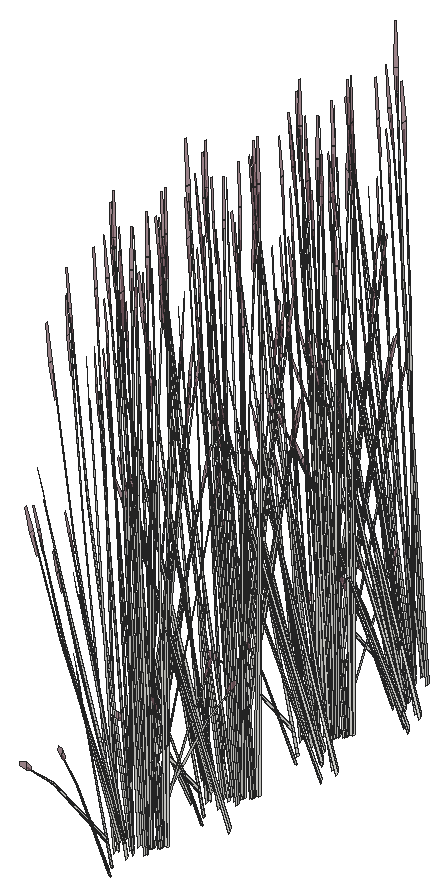
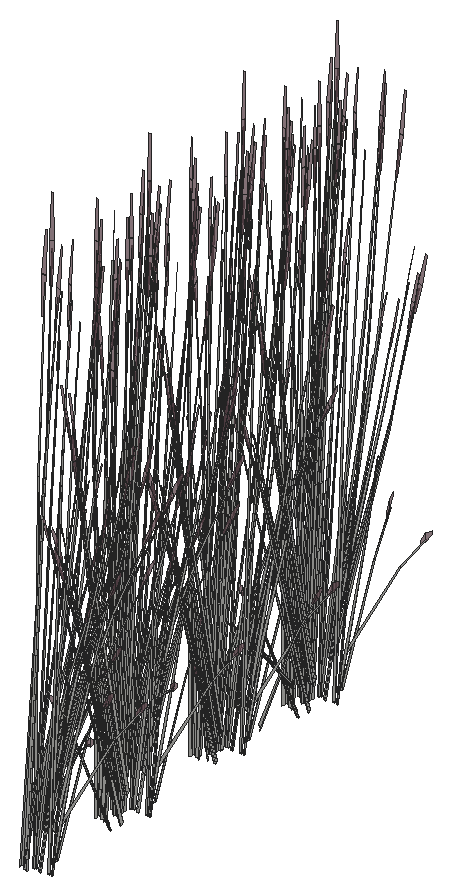
# SketchUp Ruby script. Lengths in inches.
U = 1.inch
M = Sketchup.active_model
def pt(a) = Geom::Point3d.new(a.map { |v| v * U })
def face(e, loops, mat)
  f = e.add_face(loops[0].map { |a| pt(a) })
  loops[1..].each { |l| e.add_face(l.map { |a| pt(a) }).erase! }
  f.material = f.back_material = mat if mat
  f
end
# faces: each face lists its corners as indices into pts; further lists are holes
def faces(e, pts, list, mat = nil) = list.each { |f| face(e, (f[0].is_a?(Array) ? f : [f]).map { |l| l.map { |i| pts[i] } }, mat) }
# xy, xz, yz: faces in a plane at the given z, y or x. An outline is a flat list of corners, or four numbers for a rectangle; further outlines are holes
def ring(l) = l.size == 4 ? [[l[0], l[1]], [l[2], l[1]], [l[2], l[3]], [l[0], l[3]]] : l.each_slice(2).to_a
def flat(e, list, mat, &to3) = list.each { |f| face(e, (f[0].is_a?(Array) ? f : [f]).map { |l| ring(l).map { |u, v| to3.(u, v) } }, mat) }
def xy(e, z, list, mat = nil) = flat(e, list, mat) { |x, y| [x, y, z] }
def xz(e, y, list, mat = nil) = flat(e, list, mat) { |x, z| [x, y, z] }
def yz(e, x, list, mat = nil) = flat(e, list, mat) { |y, z| [x, y, z] }
def lines(e, pts, list) = list.each { |a, b| e.add_line(pt(pts[a]), pt(pts[b])) }
# prism: a flat outline (further loops are holes) pulled along v
def prism(e, loops, v, mat = nil)
  f = face(e, loops, mat); d = Geom::Vector3d.new(v.map { |x| x * U })
  f.pushpull(f.normal.samedirection?(d) ? d.length : -d.length)
end
def box(e, o, s, mat = nil) = prism(e, [[o, [o[0] + s[0], o[1], o[2]], [o[0] + s[0], o[1] + s[1], o[2]], [o[0], o[1] + s[1], o[2]]]], [0, 0, s[2]], mat)
def at(x, y, z, deg = 0) = Geom::Transformation.translation(pt([x, y, z])) * Geom::Transformation.rotation(ORIGIN, Z_AXIS, deg.degrees)
def axes(o, x, y, z) = Geom::Transformation.new([*x, 0, *y, 0, *z, 0, *pt(o).to_a, 1])
def part(name) = M.definitions.add(name)
# library, detail: a bought-in or finely detailed component or shape, given as its bounding box
def library(name, o, s) = part(name).tap { |d| box(d.entities, o, s) }
def detail(e, o, s) = box(e.add_group.entities, o, s)
def put(e, d, t, mat = nil) = e.add_instance(d, t).tap { |i| i.material = mat if mat }
def group(e, t, mat = nil) = e.add_group.tap { |g| g.transformation = t; g.material = mat if mat }.entities
root = M.entities
M.materials.add("LightPink_Translucent").color = [144, 107, 117]
M.materials["LightPink_Translucent"].alpha = 0.75
c1 = part("blade")
p = [[2.15,0.21,22],[0,0.17,0],[0.09,0.45,0],[2.18,0.31,22],[2.29,0.31,22],[0.38,0.45,0],
  [2.48,0.24,33],[2.49,0.24,33],[2.48,0.22,33]]
faces(c1.entities,p,[[0,1,2,3],[4,5,2,3],[6,3,4,7],[8,0,3,6]])
c2 = part("seeds")
p = [[0.3,-0.1,1.38],[-0.01,-0.03,1.59],[-0.01,-0.03,0.03],[0.14,-0.07,-0.07],[0.29,-0.03,3],[0.15,0.01,3.11]]
faces(c2.entities,p,[[0,1,2,3],[1,0,4,5]],"LightPink_Translucent")
c3 = part("blade with seeds")
put(c3.entities,c1,at(0,0,0))
put(c3.entities,c2,axes([2.4,0.25,30.99],[1.5799,-0.05474,1.17369],[-0.12525,1.92788,0.29478],[-0.07173,-0.02425,1.56792]))
put(root,c3,axes([403.09,8.77,-7.61],[-0.07822,-0.07621,1.62908],[-0.52201,0.04832,-0.25764],[-0.08331,-0.18228,0.13065]))
put(root,c3,axes([403.63,10.06,-7.36],[-0.24409,-0.44196,-0.66157],[0.50245,-0.2463,0.07984],[-0.05708,-0.21354,0.93586]))
put(root,c3,axes([403.21,9.08,-10.61],[-0.08578,0.01958,1.6421],[-0.47437,-0.22044,-0.25086],[0.00796,-0.18387,0.2797]))
put(root,c3,axes([403.68,9.68,-7.78],[0.15418,-0.41799,-0.32977],[0.44981,0.12192,0.42575],[-0.04124,-0.16829,0.81462]))
put(root,c3,axes([403.45,9.97,-7.64],[-0.50273,-0.13626,-0.47583],[0.17232,-0.46717,-0.36857],[-0.0461,-0.18809,0.91046]))
put(root,c3,axes([403.88,9.95,-7.3125],[-0.50045,0.25306,-0.11324],[-0.24593,-0.44915,-0.62851],[-0.06603,-0.18927,0.95501]))
put(root,c3,axes([403.87,9.74,-7.6],[0.37684,-0.18473,0.05988],[0.18445,0.33686,0.47138],[-0.03639,-0.14849,0.71878]))
put(root,c3,axes([402.51,11.72,-10.05],[-0.21003,-0.55738,-0.65031],[0.60499,-0.20074,-0.17068],[-0.02321,-0.18874,1.43544]))
put(root,c3,axes([403.73,10.12,-7.3],[-0.15418,0.41799,0.32977],[-0.44981,-0.12192,-0.42575],[-0.04124,-0.16829,0.81462]))
put(root,c3,axes([403.125,9.46,-10.02],[-0.35341,0.31182,-0.03625],[-0.32382,-0.34152,-0.16435],[-0.0228,-0.09677,0.54209]))
put(root,c3,axes([401.27,11.64,-10.12],[0,-0.54355,-0.46235],[0.57217,0,0],[0,-0.1238,1.46668]))
put(root,c3,axes([402.82,11.86,-9.94],[0.24813,-0.48978,-0.41661],[0.51557,0.23571,0.2005],[0,-0.1129,1.33761]))
put(root,c3,axes([401.51,11.65,-10.11],[0.35699,-0.33913,-0.28847],[0.35699,0.33913,0.28847],[0,-0.10923,1.29413]))
put(root,c3,axes([402.76,12.27,-9.52],[-0.57594,-0.25935,-0.27094],[0.27732,-0.5474,-0.46562],[-0.0181,-0.1344,1.4872]))
put(root,c3,axes([401.51,12.14,-9.69],[0,0.54355,0.46235],[-0.57217,0,0],[0,-0.1238,1.46668]))
put(root,c3,axes([402.93,11.9375,-9.8],[0.22235,0.6078,0.42607],[-0.63531,0.21135,0.16719],[0.00776,-0.11168,1.47927]))
put(root,c3,axes([402.82,12.42,-9.47],[-0.24813,0.48978,0.41661],[-0.51557,-0.23571,-0.2005],[0,-0.1129,1.33761]))
put(root,c3,axes([403.89,12.48,-9.86],[-0.47569,-0.46784,-0.05709],[0.47598,-0.46812,0],[-0.01661,-0.01634,1.63492]))
put(root,c3,axes([402.98,12.53,-9.8],[0.64638,0.11452,0.42607],[-0.13155,0.64678,0.16719],[-0.09446,-0.06245,1.47927]))
put(root,c3,axes([402.64,13.57,-9.7],[0.54955,-0.14427,0.16428],[0.1357,0.53689,0.32672],[-0.04901,-0.07823,1.49371]))
put(root,c3,axes([403.46,13.44,-9.95],[-0.16686,-0.46861,0],[0.47648,-0.16411,0],[0,0,1.4375]))
put(root,c3,axes([403.14,13,-9.5625],[-0.09866,0.48509,0.13483],[-0.48202,-0.0842,-0.38503],[-0.08772,-0.04981,1.18024]))
put(root,c3,axes([404.27,13.6,-9.7],[0.14774,-0.54019,0.16428],[0.54062,0.15287,0.32672],[-0.09339,0.00263,1.49371]))
put(root,c3,axes([403.34,13.65,-9.95],[-0.51557,-0.24403,0],[0.24813,-0.50705,0],[0,0,1.51513]))
put(root,c3,axes([404.01,12.64,-9.47],[0.55535,-0.03355,0.41661],[0.05022,0.55698,-0.2005],[-0.09942,0.05645,1.33761]))
put(root,c3,axes([404.13,14.2,-9.96],[-0.31576,-0.54657,-0.04789],[0.53494,-0.30375,0.48057],[-0.13182,0.05204,1.52373]))
put(root,c3,axes([404.02,12.88,-9.5625],[0.37783,0.32657,0.13483],[-0.31516,0.36844,-0.38503],[-0.08772,0.04981,1.18024]))
put(root,c3,axes([404.42,13.89,-9.69],[0.47863,-0.27177,0.46235],[0.28609,0.48733,0],[-0.10901,0.0619,1.46668]))
put(root,c3,axes([403.99,14.13,-10.11],[-0.47712,-0.13449,-0.28847],[0.12013,-0.47362,0.28847],[-0.09619,0.05462,1.29413]))
put(root,c3,axes([403.91,12.76,-9.52],[0.05959,0.62022,-0.27094],[-0.62068,0.0375,-0.46562],[-0.1093,0.08261,1.4872]))
put(root,c3,axes([404.13,12.52,-9.94],[-0.24813,0.48978,-0.41661],[-0.51557,-0.23571,0.2005],[0,0.1129,1.33761]))
put(root,c3,axes([404.15,13.92,-9.83],[0.64025,0.17667,0.2864],[-0.16018,0.63149,-0.33981],[-0.10597,0.07904,1.53541]))
put(root,c3,axes([404.1,14.35,-10.12],[-0.47863,0.27177,-0.46235],[-0.28609,-0.48733,0],[-0.10901,0.0619,1.46668]))
put(root,c3,axes([403.7,19.37,-7.61],[-0.07822,-0.07621,1.62908],[-0.52201,0.04832,-0.25764],[-0.08331,-0.18228,0.13065]))
put(root,c3,axes([404.25,20.66,-7.36],[-0.24409,-0.44196,-0.66157],[0.50245,-0.2463,0.07984],[-0.05708,-0.21354,0.93586]))
put(root,c3,axes([408.66,16.62,-8.39],[0.21212,-0.01231,1.59586],[-0.14072,0.53355,0.12904],[-0.3023,-0.033,0.68222]))
put(root,c3,axes([403.83,19.68,-10.61],[-0.08578,0.01958,1.6421],[-0.47437,-0.22044,-0.25086],[0.00796,-0.18387,0.2797]))
put(root,c3,axes([401.94,13.68,-7.3],[0.34603,-0.28618,0.32977],[0.32756,0.32677,-0.42575],[-0.04984,0.16603,0.81462]))
put(root,c3,axes([404.54,14.26,-9.79],[0.31974,0.54466,0],[-0.53494,0.30375,-0.48057],[-0.12184,0.06918,1.52448]))
put(root,c3,axes([404.26,12.11,-9.35],[-0.01397,-0.51177,1.31553],[0.63227,0.13266,0.557],[-0.14954,0.28003,1.24175]))
put(root,c3,axes([404.07,20.57,-7.64],[-0.50273,-0.13626,-0.47583],[0.17232,-0.46717,-0.36857],[-0.0461,-0.18809,0.91046]))
put(root,c3,axes([403.07,20.27,-7.26],[0.56969,-0.13971,0.50064],[0.09887,0.54803,0.4128],[-0.13398,-0.16152,1.03595]))
put(root,c3,axes([404.5,20.54,-7.3125],[-0.50045,0.25306,-0.11324],[-0.24593,-0.44915,-0.62851],[-0.06603,-0.18927,0.95501]))
put(root,c3,axes([402.77,14.53,-7.6],[-0.37684,0.18473,0.05988],[-0.18445,-0.33686,0.47138],[0.03639,0.14849,0.71878]))
put(root,c3,axes([402.51,19.78,-9.42],[0.26677,0.18918,1.06958],[-0.38851,0.11372,0.78586],[-0.08313,-0.14539,0.23558]))
put(root,c3,axes([401.72,13.76,-6.97],[0.56206,0.02693,-0.12569],[-0.01536,0.50991,-0.69765],[-0.03904,0.19638,1.06006]))
put(root,c3,axes([402.91,14.5,-7.28],[-0.50393,-0.1421,0.49617],[0.17232,-0.46717,0.40911],[0.03028,0.18372,1.0267]))
put(root,c3,axes([402.85,14.43,-10.61],[0.08277,-0.02958,1.6421],[0.49786,0.16279,-0.25086],[0.01456,0.18348,0.2797]))
put(root,c3,axes([402.11,13.95,-7.34],[0.3661,0.36521,-0.52818],[-0.38674,0.31985,-0.40911],[-0.0557,0.18556,1.01061]))
put(root,c3,axes([403.2,20.39,-7.6],[0.23243,-0.34529,0.05988],[0.331,0.20103,0.47138],[-0.10701,-0.1107,0.71878]))
put(root,c3,axes([401.71,14.5,-9.37],[0.46459,-0.09625,0.0606],[0.10681,0.38778,-0.80367],[-0.02945,0.1963,0.72038]))
put(root,c3,axes([403.125,22.32,-10.05],[-0.21003,-0.55738,-0.65031],[0.60499,-0.20074,-0.17068],[-0.02321,-0.18874,1.43544]))
put(root,c3,axes([402.96,14.6,-7.78],[-0.15418,0.41799,-0.32977],[-0.44981,-0.12192,0.42575],[0.04124,0.16829,0.81462]))
put(root,c3,axes([404.35,20.72,-7.3],[-0.15418,0.41799,0.32977],[-0.44981,-0.12192,-0.42575],[-0.04124,-0.16829,0.81462]))
put(root,c3,axes([402.52,13.43,-8.39],[-0.01252,-0.20862,1.59586],[0.54251,0.1384,0.12904],[-0.03356,0.2973,0.68222]))
put(root,c3,axes([403.74,20.06,-10.02],[-0.35341,0.31182,-0.03625],[-0.32382,-0.34152,-0.16435],[-0.0228,-0.09677,0.54209]))
put(root,c3,axes([402.65,15.34,-7.61],[0.06483,0.08753,1.62908],[0.52315,0.03439,-0.25764],[0.05261,0.19303,0.13065]))
put(root,c3,axes([401.89,22.24,-10.12],[0,-0.54355,-0.46235],[0.57217,0,0],[0,-0.1238,1.46668]))
put(root,c3,axes([402.13,22.25,-10.11],[0.35699,-0.33913,-0.28847],[0.35699,0.33913,0.28847],[0,-0.10923,1.29413]))
put(root,c3,axes([403.38,22.87,-9.52],[-0.57594,-0.25935,-0.27094],[0.27732,-0.5474,-0.46562],[-0.0181,-0.1344,1.4872]))
put(root,c3,axes([403.53,23.44,-9.73],[0.13555,-0.64407,-0.21817],[0.64269,0.11227,0.47743],[-0.1123,-0.08895,1.45677]))
put(root,c3,axes([402.13,22.74,-9.69],[0,0.54355,0.46235],[-0.57217,0,0],[0,-0.1238,1.46668]))
put(root,c3,axes([403.48,23.18,-9.94],[-0.30722,-0.45622,-0.41661],[0.46535,-0.32126,0.2005],[-0.09942,-0.05645,1.33761]))
put(root,c3,axes([403.43,23.02,-9.47],[-0.24813,0.48978,0.41661],[-0.51557,-0.23571,-0.2005],[0,-0.1129,1.33761]))
put(root,c3,axes([404.51,23.08,-9.86],[-0.47569,-0.46784,-0.05709],[0.47598,-0.46812,0],[-0.01661,-0.01634,1.63492]))
put(root,c3,axes([403.6,23.13,-9.8],[0.64638,0.11452,0.42607],[-0.13155,0.64678,0.16719],[-0.09446,-0.06245,1.47927]))
put(root,c3,axes([403.25,24.17,-9.7],[0.54955,-0.14427,0.16428],[0.1357,0.53689,0.32672],[-0.04901,-0.07823,1.49371]))
put(root,c3,axes([403.76,23.59,-9.5625],[-0.09866,0.48509,0.13483],[-0.48202,-0.0842,-0.38503],[-0.08772,-0.04981,1.18024]))
put(root,c3,axes([404.89,24.2,-9.7],[0.14774,-0.54019,0.16428],[0.54062,0.15287,0.32672],[-0.09339,0.00263,1.49371]))
put(root,c3,axes([403.96,24.25,-9.95],[-0.51557,-0.24403,0],[0.24813,-0.50705,0],[0,0,1.51513]))
put(root,c3,axes([404.39,23.6,-9.7],[-0.49938,-0.43748,-0.23459],[0.42021,-0.49126,0.51337],[-0.13447,0.05118,1.56642]))
put(root,c3,axes([403.07,24.44,-9.69],[0.47863,0.27177,0.46235],[-0.28609,0.48733,0],[-0.10901,-0.0619,1.46668]))
put(root,c3,axes([404.63,23.24,-9.47],[0.55535,-0.03355,0.41661],[0.05022,0.55698,-0.2005],[-0.09942,0.05645,1.33761]))
put(root,c3,axes([404.14,23.51,-9.94],[-0.55535,0.03355,-0.41661],[-0.05022,-0.55698,0.2005],[-0.09942,0.05645,1.33761]))
put(root,c3,axes([404.75,24.8,-9.96],[-0.31576,-0.54657,-0.04789],[0.53494,-0.30375,0.48057],[-0.13182,0.05204,1.52373]))
put(root,c3,axes([404.64,23.48,-9.5625],[0.37783,0.32657,0.13483],[-0.31516,0.36844,-0.38503],[-0.08772,0.04981,1.18024]))
put(root,c3,axes([404.61,24.73,-10.11],[-0.47712,-0.13449,-0.28847],[0.12013,-0.47362,0.28847],[-0.09619,0.05462,1.29413]))
put(root,c3,axes([404.53,23.36,-9.52],[0.05959,0.62022,-0.27094],[-0.62068,0.0375,-0.46562],[-0.1093,0.08261,1.4872]))
put(root,c3,axes([404.77,24.52,-9.83],[0.64025,0.17667,0.2864],[-0.16018,0.63149,-0.33981],[-0.10597,0.07904,1.53541]))
put(root,c3,axes([404.72,24.95,-10.12],[-0.47863,0.27177,-0.46235],[-0.28609,-0.48733,0],[-0.10901,0.0619,1.46668]))
put(root,c3,axes([402.5625,24.28,-7.3],[0.34603,-0.28618,0.32977],[0.32756,0.32677,-0.42575],[-0.04984,0.16603,0.81462]))
put(root,c3,axes([405.15,24.86,-9.79],[0.31974,0.54466,0],[-0.53494,0.30375,-0.48057],[-0.12184,0.06918,1.52448]))
put(root,c3,axes([404.88,22.71,-9.35],[-0.01397,-0.51177,1.31553],[0.63227,0.13266,0.557],[-0.14954,0.28003,1.24175]))
put(root,c3,axes([407.875,28.96,-9.59],[0.09985,0.15133,1.33163],[-0.23008,0.41134,-0.28638],[-0.23625,-0.09832,0.56934]))
put(root,c3,axes([408.29,28.82,-7.36],[-0.51122,-0.01309,-0.66157],[0.03434,-0.5511,0.07984],[-0.21658,-0.05816,0.93586]))
put(root,c3,axes([403.33,31.36,-7.61],[-0.07822,-0.07621,1.62908],[-0.52201,0.04832,-0.25764],[-0.08331,-0.18228,0.13065]))
put(root,c3,axes([403.39,25.13,-7.6],[-0.37684,0.18473,0.05988],[-0.18445,-0.33686,0.47138],[0.03639,0.14849,0.71878]))
put(root,c3,axes([402.34,24.36,-6.97],[0.56206,0.02693,-0.12569],[-0.01536,0.50991,-0.69765],[-0.03904,0.19638,1.06006]))
put(root,c3,axes([403.88,32.64,-7.36],[-0.24409,-0.44196,-0.66157],[0.50245,-0.2463,0.07984],[-0.05708,-0.21354,0.93586]))
put(root,c3,axes([403.53,25.1,-7.28],[-0.50393,-0.1421,0.49617],[0.17232,-0.46717,0.40911],[0.03028,0.18372,1.0267]))
put(root,c3,axes([402.6,25.8,-9.42],[-0.01324,-0.32319,1.06958],[0.33072,0.23052,0.78586],[-0.06504,0.15405,0.23558]))
put(root,c3,axes([403.46,31.66,-10.61],[-0.08578,0.01958,1.6421],[-0.47437,-0.22044,-0.25086],[0.00796,-0.18387,0.2797]))
put(root,c3,axes([402.73,24.55,-7.34],[0.3661,0.36521,-0.52818],[-0.38674,0.31985,-0.40911],[-0.0557,0.18556,1.01061]))
put(root,c3,axes([402.33,25.1,-9.37],[0.46459,-0.09625,0.0606],[0.10681,0.38778,-0.80367],[-0.02945,0.1963,0.72038]))
put(root,c3,axes([403.92,32.27,-7.78],[0.15418,-0.41799,-0.32977],[0.44981,0.12192,0.42575],[-0.04124,-0.16829,0.81462]))
put(root,c3,axes([407.65,29.32,-8.39],[0.21212,-0.01231,1.59586],[-0.14072,0.53355,0.12904],[-0.3023,-0.033,0.68222]))
put(root,c3,axes([403.69,32.55,-7.64],[-0.50273,-0.13626,-0.47583],[0.17232,-0.46717,-0.36857],[-0.0461,-0.18809,0.91046]))
put(root,c3,axes([402.61,24.39,-7.03],[-0.01331,0.50278,-0.73435],[-0.56035,-0.03377,0.08862],[-0.05914,0.213,1.03881]))
put(root,c3,axes([403.14,24.03,-8.39],[-0.01252,-0.20862,1.59586],[0.54251,0.1384,0.12904],[-0.03356,0.2973,0.68222]))
put(root,c3,axes([404.125,32.53,-7.3125],[-0.50045,0.25306,-0.11324],[-0.24593,-0.44915,-0.62851],[-0.06603,-0.18927,0.95501]))
put(root,c3,axes([402.75,34.3,-10.05],[-0.21003,-0.55738,-0.65031],[0.60499,-0.20074,-0.17068],[-0.02321,-0.18874,1.43544]))
put(root,c3,axes([402.42,25.09,-8.87],[0.01124,-0.2806,1.43727],[0.50537,0.14821,0.19862],[-0.04379,0.29905,0.67868]))
put(root,c3,axes([407.47,29.78,-7.78],[-0.42502,-0.15163,-0.32977],[0.12396,-0.44238,0.42575],[-0.17112,0.04056,0.81462]))
put(root,c3,axes([403.97,32.71,-7.3],[-0.15418,0.41799,0.32977],[-0.44981,-0.12192,-0.42575],[-0.04124,-0.16829,0.81462]))
put(root,c3,axes([403.37,32.04,-10.02],[-0.35341,0.31182,-0.03625],[-0.32382,-0.34152,-0.16435],[-0.0228,-0.09677,0.54209]))
put(root,c3,axes([408.76,29.7,-8.89],[0.14537,-0.07863,1.64882],[0.05013,0.549,0.12904],[-0.31487,0.07285,0.5893]))
put(root,c3,axes([401.51,34.22,-10.12],[0,-0.54355,-0.46235],[0.57217,0,0],[0,-0.1238,1.46668]))
put(root,c3,axes([407.2,30.07,-7.61],[-0.08351,0.07057,1.62908],[0.0071,0.51561,-0.25764],[-0.19143,0.06705,0.13065]))
put(root,c3,axes([403.07,34.45,-9.94],[0.24813,-0.48978,-0.41661],[0.51557,0.23571,0.2005],[0,-0.1129,1.33761]))
put(root,c3,axes([401.76,34.24,-10.11],[0.35699,-0.33913,-0.28847],[0.35699,0.33913,0.28847],[0,-0.10923,1.29413]))
put(root,c3,axes([403.01,34.85,-9.52],[-0.57594,-0.25935,-0.27094],[0.27732,-0.5474,-0.46562],[-0.0181,-0.1344,1.4872]))
put(root,c3,axes([407.74,30.26,-8.39],[0.17745,-0.11497,1.59586],[0.14939,0.53127,0.12904],[-0.27857,0.12007,0.68222]))
put(root,c3,axes([407.19,31.16,-9.59],[0.17773,0.04462,1.33163],[0.11455,0.45576,-0.28638],[-0.24142,0.08531,0.56934]))
put(root,c3,axes([403.15,35.43,-9.73],[0.13555,-0.64407,-0.21817],[0.64269,0.11227,0.47743],[-0.1123,-0.08895,1.45677]))
put(root,c3,axes([401.76,34.73,-9.69],[0,0.54355,0.46235],[-0.57217,0,0],[0,-0.1238,1.46668]))
put(root,c3,axes([403.17,34.52,-9.8],[0.22235,0.6078,0.42607],[-0.63531,0.21135,0.16719],[0.00776,-0.11168,1.47927]))
put(root,c3,axes([403.06,35,-9.47],[-0.24813,0.48978,0.41661],[-0.51557,-0.23571,-0.2005],[0,-0.1129,1.33761]))
put(root,c3,axes([404.13,35.0625,-9.86],[-0.47569,-0.46784,-0.05709],[0.47598,-0.46812,0],[-0.01661,-0.01634,1.63492]))
put(root,c3,axes([403.23,35.12,-9.8],[0.64638,0.11452,0.42607],[-0.13155,0.64678,0.16719],[-0.09446,-0.06245,1.47927]))
put(root,c3,axes([402.88,36.15,-9.7],[0.54955,-0.14427,0.16428],[0.1357,0.53689,0.32672],[-0.04901,-0.07823,1.49371]))
put(root,c3,axes([403.7,36.03,-9.95],[-0.16686,-0.46861,0],[0.47648,-0.16411,0],[0,0,1.4375]))
put(root,c3,axes([403.39,35.58,-9.5625],[-0.09866,0.48509,0.13483],[-0.48202,-0.0842,-0.38503],[-0.08772,-0.04981,1.18024]))
put(root,c3,axes([404.51,36.18,-9.7],[0.14774,-0.54019,0.16428],[0.54062,0.15287,0.32672],[-0.09339,0.00263,1.49371]))
put(root,c3,axes([403.59,36.24,-9.95],[-0.51557,-0.24403,0],[0.24813,-0.50705,0],[0,0,1.51513]))
put(root,c3,axes([402.7,36.43,-9.69],[0.47863,0.27177,0.46235],[-0.28609,0.48733,0],[-0.10901,-0.0619,1.46668]))
put(root,c3,axes([407.58,39.29,-8.39],[0.18996,0.09365,1.59586],[-0.39312,0.39287,0.12904],[-0.24502,-0.17723,0.68222]))
put(root,c3,axes([404.26,35.23,-9.47],[0.55535,-0.03355,0.41661],[0.05022,0.55698,-0.2005],[-0.09942,0.05645,1.33761]))
put(root,c3,axes([404.375,36.79,-9.96],[-0.31576,-0.54657,-0.04789],[0.53494,-0.30375,0.48057],[-0.13182,0.05204,1.52373]))
put(root,c3,axes([404.26,35.47,-9.5625],[0.37783,0.32657,0.13483],[-0.31516,0.36844,-0.38503],[-0.08772,0.04981,1.18024]))
put(root,c3,axes([404.67,36.47,-9.69],[0.47863,-0.27177,0.46235],[0.28609,0.48733,0],[-0.10901,0.0619,1.46668]))
put(root,c3,axes([404.23,36.72,-10.11],[-0.47712,-0.13449,-0.28847],[0.12013,-0.47362,0.28847],[-0.09619,0.05462,1.29413]))
put(root,c3,axes([404.15,35.34,-9.52],[0.05959,0.62022,-0.27094],[-0.62068,0.0375,-0.46562],[-0.1093,0.08261,1.4872]))
put(root,c3,axes([407.4,39.78,-9.59],[0.09985,0.15133,1.33163],[-0.23008,0.41134,-0.28638],[-0.23625,-0.09832,0.56934]))
put(root,c3,axes([404.39,36.51,-9.83],[0.64025,0.17667,0.2864],[-0.16018,0.63149,-0.33981],[-0.10597,0.07904,1.53541]))
put(root,c3,axes([404.34,36.93,-10.12],[-0.47863,0.27177,-0.46235],[-0.28609,-0.48733,0],[-0.10901,0.0619,1.46668]))
put(root,c3,axes([407.8125,39.65,-7.36],[-0.51122,-0.01309,-0.66157],[0.03434,-0.5511,0.07984],[-0.21658,-0.05816,0.93586]))
put(root,c3,axes([402.1875,36.27,-7.3],[0.34603,-0.28618,0.32977],[0.32756,0.32677,-0.42575],[-0.04984,0.16603,0.81462]))
put(root,c3,axes([404.78,36.85,-9.79],[0.31974,0.54466,0],[-0.53494,0.30375,-0.48057],[-0.12184,0.06918,1.52448]))
put(root,c3,axes([407.12,38.75,-7.62],[0.03791,0.05424,1.65179],[-0.18278,0.48761,-0.15608],[-0.18511,0.00353,0.29231]))
put(root,c3,axes([404.51,34.69,-9.35],[-0.01397,-0.51177,1.31553],[0.63227,0.13266,0.557],[-0.14954,0.28003,1.24175]))
put(root,c3,axes([407.64,39.76,-7.64],[-0.37135,0.36005,-0.47583],[-0.32522,-0.38035,-0.36857],[-0.18868,-0.05478,0.91046]))
put(root,c3,axes([407.18,40.15,-8.39],[0.21212,-0.01231,1.59586],[-0.14072,0.53355,0.12904],[-0.3023,-0.033,0.68222]))
put(root,c3,axes([403.35,43.21,-7.61],[-0.07822,-0.07621,1.62908],[-0.52201,0.04832,-0.25764],[-0.08331,-0.18228,0.13065]))
put(root,c3,axes([403.9,44.5,-7.36],[-0.24409,-0.44196,-0.66157],[0.50245,-0.2463,0.07984],[-0.05708,-0.21354,0.93586]))
put(root,c3,axes([403.02,37.12,-7.6],[-0.37684,0.18473,0.05988],[-0.18445,-0.33686,0.47138],[0.03639,0.14849,0.71878]))
put(root,c3,axes([401.97,36.35,-6.97],[0.56206,0.02693,-0.12569],[-0.01536,0.50991,-0.69765],[-0.03904,0.19638,1.06006]))
put(root,c3,axes([403.15,37.08,-7.28],[-0.50393,-0.1421,0.49617],[0.17232,-0.46717,0.40911],[0.03028,0.18372,1.0267]))
put(root,c3,axes([403.48,43.52,-10.61],[-0.08578,0.01958,1.6421],[-0.47437,-0.22044,-0.25086],[0.00796,-0.18387,0.2797]))
put(root,c3,axes([403.1,37.01,-10.61],[0.08277,-0.02958,1.6421],[0.49786,0.16279,-0.25086],[0.01456,0.18348,0.2797]))
put(root,c3,axes([402.35,36.54,-7.34],[0.3661,0.36521,-0.52818],[-0.38674,0.31985,-0.40911],[-0.0557,0.18556,1.01061]))
put(root,c3,axes([403.95,44.125,-7.78],[0.15418,-0.41799,-0.32977],[0.44981,0.12192,0.42575],[-0.04124,-0.16829,0.81462]))
put(root,c3,axes([401.95,37.09,-9.37],[0.46459,-0.09625,0.0606],[0.10681,0.38778,-0.80367],[-0.02945,0.1963,0.72038]))
put(root,c3,axes([407.04,40.8,-10.61],[0.01297,0.08566,1.6421],[-0.26146,0.44735,-0.25086],[-0.18572,-0.02255,0.2797]))
put(root,c3,axes([403.72,44.41,-7.64],[-0.50273,-0.13626,-0.47583],[0.17232,-0.46717,-0.36857],[-0.0461,-0.18809,0.91046]))
put(root,c3,axes([403.21,37.18,-7.78],[-0.15418,0.41799,-0.32977],[-0.44981,-0.12192,0.42575],[0.04124,0.16829,0.81462]))
put(root,c3,axes([406.99,40.6,-7.78],[-0.42502,-0.15163,-0.32977],[0.12396,-0.44238,0.42575],[-0.17112,0.04056,0.81462]))
put(root,c3,axes([402.77,36.02,-8.39],[-0.01252,-0.20862,1.59586],[0.54251,0.1384,0.12904],[-0.03356,0.2973,0.68222]))
put(root,c3,axes([404.15,44.39,-7.3125],[-0.50045,0.25306,-0.11324],[-0.24593,-0.44915,-0.62851],[-0.06603,-0.18927,0.95501]))
put(root,c3,axes([402.84,44.24,-7.6],[0.23243,-0.34529,0.05988],[0.331,0.20103,0.47138],[-0.10701,-0.1107,0.71878]))
put(root,c3,axes([408.29,40.53,-8.89],[0.14537,-0.07863,1.64882],[0.05013,0.549,0.12904],[-0.31487,0.07285,0.5893]))
put(root,c3,axes([402.77,46.16,-10.05],[-0.21003,-0.55738,-0.65031],[0.60499,-0.20074,-0.17068],[-0.02321,-0.18874,1.43544]))
put(root,c3,axes([404,44.57,-7.3],[-0.15418,0.41799,0.32977],[-0.44981,-0.12192,-0.42575],[-0.04124,-0.16829,0.81462]))
put(root,c3,axes([402.05,37.08,-8.87],[0.01124,-0.2806,1.43727],[0.50537,0.14821,0.19862],[-0.04379,0.29905,0.67868]))
put(root,c3,axes([406.72,40.9,-7.61],[-0.08351,0.07057,1.62908],[0.0071,0.51561,-0.25764],[-0.19143,0.06705,0.13065]))
put(root,c3,axes([407.28,40.83,-7.64],[-0.13855,0.49442,-0.47583],[-0.47502,-0.16947,-0.36857],[-0.19125,0.04534,0.91046]))
put(root,c3,axes([403.39,43.9,-10.02],[-0.35341,0.31182,-0.03625],[-0.32382,-0.34152,-0.16435],[-0.0228,-0.09677,0.54209]))
put(root,c3,axes([401.53,46.08,-10.12],[0,-0.54355,-0.46235],[0.57217,0,0],[0,-0.1238,1.46668]))
put(root,c3,axes([407.27,41.09,-8.39],[0.17745,-0.11497,1.59586],[0.14939,0.53127,0.12904],[-0.27857,0.12007,0.68222]))
put(root,c3,axes([403.09,46.3,-9.94],[0.24813,-0.48978,-0.41661],[0.51557,0.23571,0.2005],[0,-0.1129,1.33761]))
put(root,c3,axes([406.71,41.99,-9.59],[0.17773,0.04462,1.33163],[0.11455,0.45576,-0.28638],[-0.24142,0.08531,0.56934]))
put(root,c3,axes([401.78,46.1,-10.11],[0.35699,-0.33913,-0.28847],[0.35699,0.33913,0.28847],[0,-0.10923,1.29413]))
put(root,c3,axes([403.03,46.71,-9.52],[-0.57594,-0.25935,-0.27094],[0.27732,-0.5474,-0.46562],[-0.0181,-0.1344,1.4872]))
put(root,c3,axes([405.8,41.42,-7.62],[0.06527,0.01458,1.65179],[0.20191,0.48025,-0.15608],[-0.1336,0.12605,0.29231]))
put(root,c3,axes([403.17,47.29,-9.73],[0.13555,-0.64407,-0.21817],[0.64269,0.11227,0.47743],[-0.1123,-0.08895,1.45677]))
put(root,c3,axes([401.78,46.59,-9.69],[0,0.54355,0.46235],[-0.57217,0,0],[0,-0.1238,1.46668]))
put(root,c3,axes([403.19,46.38,-9.8],[0.22235,0.6078,0.42607],[-0.63531,0.21135,0.16719],[0.00776,-0.11168,1.47927]))
put(root,c3,axes([403.08,46.86,-9.47],[-0.24813,0.48978,0.41661],[-0.51557,-0.23571,-0.2005],[0,-0.1129,1.33761]))
put(root,c3,axes([404.15,46.92,-9.86],[-0.47569,-0.46784,-0.05709],[0.47598,-0.46812,0],[-0.01661,-0.01634,1.63492]))
put(root,c3,axes([403.25,46.98,-9.8],[0.64638,0.11452,0.42607],[-0.13155,0.64678,0.16719],[-0.09446,-0.06245,1.47927]))
